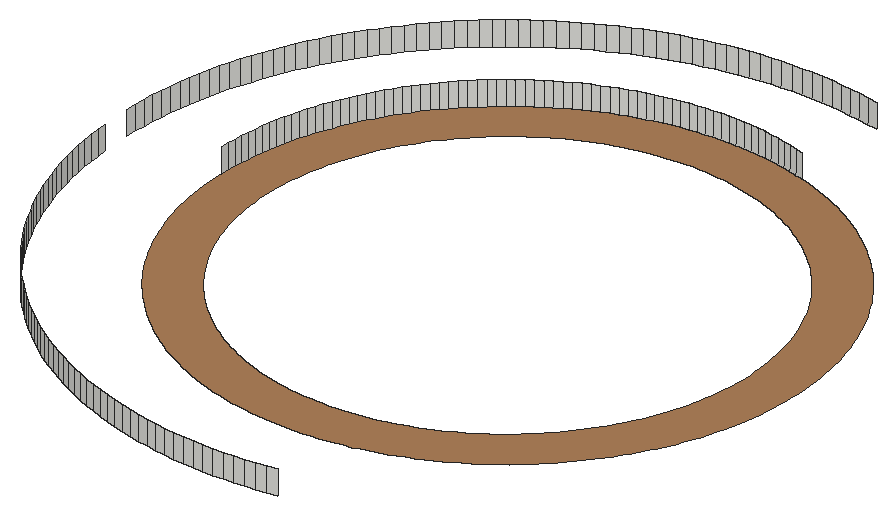
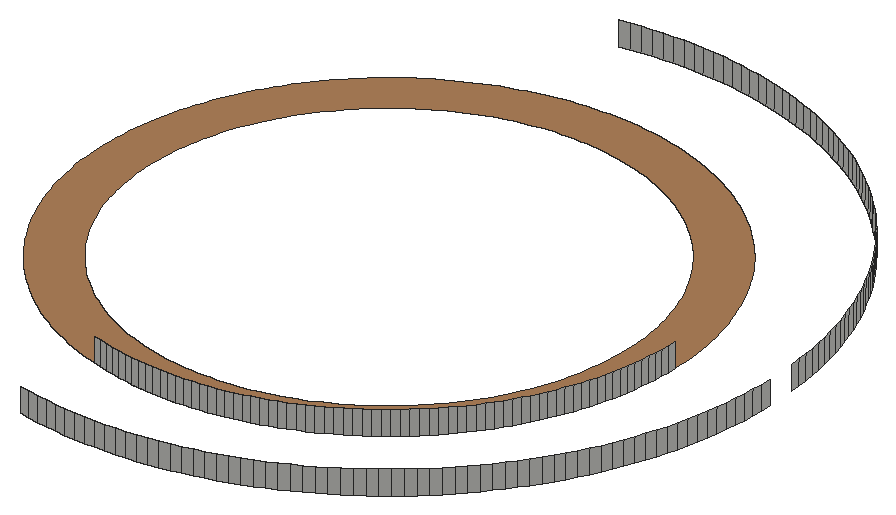
# SketchUp Ruby script. Lengths in inches.
U = 1.inch
M = Sketchup.active_model
def pt(a) = Geom::Point3d.new(a.map { |v| v * U })
def face(e, loops, mat)
  f = e.add_face(loops[0].map { |a| pt(a) })
  loops[1..].each { |l| e.add_face(l.map { |a| pt(a) }).erase! }
  f.material = f.back_material = mat if mat
  f
end
# faces: each face lists its corners as indices into pts; further lists are holes
def faces(e, pts, list, mat = nil) = list.each { |f| face(e, (f[0].is_a?(Array) ? f : [f]).map { |l| l.map { |i| pts[i] } }, mat) }
# xy, xz, yz: faces in a plane at the given z, y or x. An outline is a flat list of corners, or four numbers for a rectangle; further outlines are holes
def ring(l) = l.size == 4 ? [[l[0], l[1]], [l[2], l[1]], [l[2], l[3]], [l[0], l[3]]] : l.each_slice(2).to_a
def flat(e, list, mat, &to3) = list.each { |f| face(e, (f[0].is_a?(Array) ? f : [f]).map { |l| ring(l).map { |u, v| to3.(u, v) } }, mat) }
def xy(e, z, list, mat = nil) = flat(e, list, mat) { |x, y| [x, y, z] }
def xz(e, y, list, mat = nil) = flat(e, list, mat) { |x, z| [x, y, z] }
def yz(e, x, list, mat = nil) = flat(e, list, mat) { |y, z| [x, y, z] }
def lines(e, pts, list) = list.each { |a, b| e.add_line(pt(pts[a]), pt(pts[b])) }
# prism: a flat outline (further loops are holes) pulled along v
def prism(e, loops, v, mat = nil)
  f = face(e, loops, mat); d = Geom::Vector3d.new(v.map { |x| x * U })
  f.pushpull(f.normal.samedirection?(d) ? d.length : -d.length)
end
def box(e, o, s, mat = nil) = prism(e, [[o, [o[0] + s[0], o[1], o[2]], [o[0] + s[0], o[1] + s[1], o[2]], [o[0], o[1] + s[1], o[2]]]], [0, 0, s[2]], mat)
def at(x, y, z, deg = 0) = Geom::Transformation.translation(pt([x, y, z])) * Geom::Transformation.rotation(ORIGIN, Z_AXIS, deg.degrees)
def axes(o, x, y, z) = Geom::Transformation.new([*x, 0, *y, 0, *z, 0, *pt(o).to_a, 1])
def part(name) = M.definitions.add(name)
# library, detail: a bought-in or finely detailed component or shape, given as its bounding box
def library(name, o, s) = part(name).tap { |d| box(d.entities, o, s) }
def detail(e, o, s) = box(e.add_group.entities, o, s)
def put(e, d, t, mat = nil) = e.add_instance(d, t).tap { |i| i.material = mat if mat }
def group(e, t, mat = nil) = e.add_group.tap { |g| g.transformation = t; g.material = mat if mat }.entities
root = M.entities
M.materials.add("01 - Default1").color = [173, 128, 89]
xy(root,111.3125,[[[905.98,253.26,904.09,253.28,902.21,253.35,900.33,253.48,898.45,253.65,896.58,253.87,894.72,254.14,892.86,254.46,891.01,254.83,889.17,255.25,887.34,255.71,885.53,256.22,883.73,256.78,881.94,257.39,880.18,258.04,878.43,258.74,876.69,259.48,874.98,260.27,873.29,261.1,871.625,261.98,869.98,262.9,868.36,263.87,866.76,264.87,865.2,265.92,863.66,267.01,862.15,268.13,860.67,269.3,859.22,270.51,857.8,271.75,856.42,273.03,855.07,274.34,853.75,275.69,852.47,277.08,851.23,278.5,850.02,279.95,848.86,281.43,847.73,282.9375,846.64,284.47,845.59,286.04,844.59,287.64,843.625,289.26,842.7,290.9,841.83,292.57,840.99,294.26,840.2,295.97,839.46,297.7,838.76,299.45,838.11,301.22,837.5,303.01,836.94,304.81,836.43,306.62,835.97,308.45,835.55,310.29,835.18,312.14,834.87,313.99,834.59,315.86,834.375,317.73,834.2,319.61,834.08,321.49,834,323.37,833.98,325.26,834,327.14,834.08,329.02,834.2,330.91,834.375,332.78,834.59,334.65,834.87,336.52,835.18,338.38,835.55,340.23,835.97,342.0625,836.43,343.89,836.94,345.71,837.5,347.51,838.11,349.29,838.76,351.06,839.46,352.81,840.2,354.54,840.99,356.25,841.83,357.94,842.7,359.61,843.625,361.26,844.59,362.875,845.59,364.47,846.64,366.04,847.73,367.58,848.86,369.09,850.02,370.57,851.23,372.02,852.47,373.43,853.75,374.82,855.07,376.17,856.42,377.48,857.8,378.76,859.22,380.01,860.67,381.21,862.15,382.38,863.66,383.51,865.2,384.59,866.76,385.64,868.36,386.65,869.98,387.61,871.625,388.53,873.29,389.41,874.98,390.24,876.69,391.03,878.43,391.78,880.18,392.47,881.94,393.125,883.73,393.73,885.53,394.29,887.34,394.8,889.17,395.27,891.01,395.68,892.86,396.05,894.72,396.37,896.58,396.64,898.45,396.86,900.33,397.03,902.21,397.16,904.09,397.23,905.98,397.26,907.86,397.23,909.75,397.16,911.63,397.03,913.5,396.86,915.375,396.64,917.24,396.37,919.1,396.05,920.95,395.68,922.79,395.27,924.61,394.8,926.43,394.29,928.23,393.73,930.01,393.125,931.78,392.47,933.53,391.78,935.26,391.03,936.98,390.24,938.67,389.41,940.33,388.53,941.98,387.61,943.6,386.65,945.19,385.64,946.76,384.59,948.3,383.51,949.81,382.38,951.29,381.21,952.74,380.01,954.16,378.76,955.54,377.48,956.89,376.17,958.21,374.82,959.49,373.43,960.73,372.02,961.93,370.57,963.1,369.09,964.23,367.58,965.32,366.04,966.36,364.47,967.37,362.875,968.33,361.26,969.25,359.61,970.13,357.94,970.96,356.25,971.75,354.54,972.5,352.81,973.2,351.06,973.85,349.29,974.45,347.51,975.01,345.71,975.53,343.89,975.99,342.0625,976.41,340.23,976.77,338.38,977.09,336.52,977.36,334.65,977.58,332.78,977.76,330.91,977.88,329.02,977.95,327.14,977.98,325.26,977.95,323.37,977.88,321.49,977.76,319.61,977.58,317.73,977.36,315.86,977.09,313.99,976.77,312.14,976.41,310.29,975.99,308.45,975.53,306.62,975.01,304.81,974.45,303.01,973.85,301.22,973.2,299.45,972.5,297.7,971.75,295.97,970.96,294.26,970.13,292.57,969.25,290.9,968.33,289.26,967.37,287.64,966.36,286.04,965.32,284.47,964.23,282.9375,963.1,281.43,961.93,279.95,960.73,278.5,959.49,277.08,958.21,275.69,956.89,274.34,955.54,273.03,954.16,271.75,952.74,270.51,951.29,269.3,949.81,268.13,948.3,267.01,946.76,265.92,945.19,264.87,943.6,263.87,941.98,262.9,940.33,261.98,938.67,261.1,936.98,260.27,935.26,259.48,933.53,258.74,931.78,258.04,930.01,257.39,928.23,256.78,926.43,256.22,924.61,255.71,922.79,255.25,920.95,254.83,919.1,254.46,917.24,254.14,915.375,253.87,913.5,253.65,911.63,253.48,909.75,253.35,907.86,253.28],[905.98,265.26,907.55,265.28,909.12,265.34,910.6875,265.44,912.25,265.58,913.81,265.77,915.36,265.99,916.91,266.26,918.45,266.57,919.99,266.91,921.51,267.3,923.02,267.73,924.52,268.19,926.01,268.7,927.48,269.24,928.94,269.82,930.38,270.44,931.81,271.1,933.22,271.8,934.61,272.53,935.98,273.29,937.33,274.1,938.66,274.9375,939.96,275.81,941.25,276.72,942.5,277.66,943.74,278.63,944.95,279.63,946.125,280.67,947.28,281.73,948.41,282.83,949.5,283.95,950.57,285.11,951.6,286.29,952.61,287.5,953.58,288.73,954.52,289.99,955.43,291.27,956.3,292.58,957.14,293.91,957.94,295.26,958.71,296.625,959.4375,298.02,960.13,299.43,960.79,300.85,961.41,302.3,961.99,303.75,962.54,305.23,963.04,306.72,963.51,308.22,963.93,309.73,964.32,311.25,964.67,312.78,964.97,314.32,965.24,315.87,965.47,317.42,965.65,318.98,965.79,320.55,965.9,322.12,965.96,323.6875,965.98,325.26,965.96,326.83,965.9,328.4,965.79,329.96,965.65,331.53,965.47,333.09,965.24,334.64,964.97,336.19,964.67,337.73,964.32,339.26,963.93,340.79,963.51,342.3,963.04,343.8,962.54,345.28,961.99,346.76,961.41,348.22,960.79,349.66,960.13,351.09,959.4375,352.5,958.71,353.89,957.94,355.26,957.14,356.61,956.3,357.93,955.43,359.24,954.52,360.52,953.58,361.78,952.61,363.02,951.6,364.22,950.57,365.4,949.5,366.56,948.41,367.68,947.28,368.78,946.125,369.84,944.95,370.88,943.74,371.88,942.5,372.86,941.25,373.8,939.96,374.7,938.66,375.58,937.33,376.41,935.98,377.22,934.61,377.99,933.22,378.72,931.81,379.41,930.38,380.07,928.94,380.6875,927.48,381.27,926.01,381.81,924.52,382.32,923.02,382.79,921.51,383.21,919.99,383.6,918.45,383.95,916.91,384.25,915.36,384.52,913.81,384.74,912.25,384.93,910.6875,385.07,909.12,385.17,907.55,385.24,905.98,385.26,904.41,385.24,902.84,385.17,901.27,385.07,899.71,384.93,898.15,384.74,896.59,384.52,895.04,384.25,893.5,383.95,891.97,383.6,890.45,383.21,888.9375,382.79,887.4375,382.32,885.95,381.81,884.48,381.27,883.02,380.6875,881.57,380.07,880.15,379.41,878.74,378.72,877.35,377.99,875.98,377.22,874.63,376.41,873.3,375.58,871.99,374.7,870.71,373.8,869.45,372.86,868.22,371.88,867.01,370.88,865.83,369.84,864.68,368.78,863.55,367.68,862.46,366.56,861.39,365.4,860.35,364.22,859.35,363.02,858.38,361.78,857.4375,360.52,856.53,359.24,855.66,357.93,854.82,356.61,854.02,355.26,853.25,353.89,852.52,352.5,851.82,351.09,851.17,349.66,850.55,348.22,849.96,346.76,849.42,345.28,848.92,343.8,848.45,342.3,848.02,340.79,847.64,339.26,847.29,337.73,846.98,336.19,846.72,334.64,846.49,333.09,846.31,331.53,846.16,329.96,846.0625,328.4,846,326.83,845.98,325.26,846,323.6875,846.0625,322.12,846.16,320.55,846.31,318.98,846.49,317.42,846.72,315.87,846.98,314.32,847.29,312.78,847.64,311.25,848.02,309.73,848.45,308.22,848.92,306.72,849.42,305.23,849.96,303.75,850.55,302.3,851.17,300.85,851.82,299.43,852.52,298.02,853.25,296.625,854.02,295.26,854.82,293.91,855.66,292.58,856.53,291.27,857.4375,289.99,858.38,288.73,859.35,287.5,860.35,286.29,861.39,285.11,862.46,283.95,863.55,282.83,864.68,281.73,865.83,280.67,867.01,279.63,868.22,278.63,869.45,277.66,870.71,276.72,871.99,275.81,873.3,274.9375,874.63,274.1,875.98,273.29,877.35,272.53,878.74,271.8,880.15,271.1,881.57,270.44,883.02,269.82,884.48,269.24,885.95,268.7,887.4375,268.19,888.9375,267.73,890.45,267.3,891.97,266.91,893.5,266.57,895.04,266.26,896.59,265.99,898.15,265.77,899.71,265.58,901.27,265.44,902.84,265.34,904.41,265.28]]],"01 - Default1")
p = [[900.95,229.39,117.3125],[903.47,229.29,117.3125],[903.47,229.29,111.3125],[900.95,229.39,111.3125],[905.98,229.26,117.3125],[905.98,229.26,111.3125],
  [908.49,229.29,117.3125],[908.49,229.29,111.3125],[911,229.39,117.3125],[911,229.39,111.3125],[898.45,229.55,117.3125],[898.45,229.55,111.3125],
  [913.51,229.55,117.3125],[913.51,229.55,111.3125],[895.94,229.78,117.3125],[895.94,229.78,111.3125],[916.01,229.78,117.3125],[916.01,229.78,111.3125],
  [893.45,230.08,117.3125],[893.45,230.08,111.3125],[918.51,230.08,117.3125],[918.51,230.08,111.3125],[890.96,230.4375,117.3125],[890.96,230.4375,111.3125],
  [921,230.4375,117.3125],[921,230.4375,111.3125],[888.48,230.86,117.3125],[888.48,230.86,111.3125],[923.47,230.86,117.3125],[923.47,230.86,111.3125],
  [886.02,231.35,117.3125],[886.02,231.35,111.3125],[883.57,231.91,117.3125],[883.57,231.91,111.3125],[881.13,232.53,117.3125],[881.13,232.53,111.3125],
  [878.71,233.21,117.3125],[878.71,233.21,111.3125],[876.3125,233.95,117.3125],[876.3125,233.95,111.3125],[873.93,234.76,117.3125],[873.93,234.76,111.3125],
  [871.58,235.63,117.3125],[871.58,235.63,111.3125],[869.24,236.5625,117.3125],[869.24,236.5625,111.3125],[866.93,237.56,117.3125],[866.93,237.56,111.3125],
  [864.65,238.61,117.3125],[864.65,238.61,111.3125],[862.4,239.72,117.3125],[862.4,239.72,111.3125],[860.17,240.89,117.3125],[860.17,240.89,111.3125],
  [857.98,242.12,117.3125],[857.98,242.12,111.3125],[855.82,243.4,117.3125],[855.82,243.4,111.3125],[853.69,244.74,117.3125],[853.69,244.74,111.3125],
  [851.6,246.14,117.3125],[851.6,246.14,111.3125],[849.55,247.59,117.3125],[849.55,247.59,111.3125],[847.54,249.09,117.3125],[847.54,249.09,111.3125],
  [845.5625,250.65,117.3125],[845.5625,250.65,111.3125],[843.63,252.26,117.3125],[843.63,252.26,111.3125],[841.74,253.91,117.3125],[841.74,253.91,111.3125],
  [839.9,255.62,117.3125],[839.9,255.62,111.3125],[838.1,257.375,117.3125],[838.1,257.375,111.3125],[836.34,259.17,117.3125],[836.34,259.17,111.3125],
  [834.64,261.02,117.3125],[834.64,261.02,111.3125],[832.98,262.91,117.3125],[832.98,262.91,111.3125],[831.37,264.84,117.3125],[831.37,264.84,111.3125],
  [829.82,266.82,117.3125],[829.82,266.82,111.3125],[828.3125,268.83,117.3125],[828.3125,268.83,111.3125],[826.86,270.88,117.3125],[826.86,270.88,111.3125],
  [825.47,272.97,117.3125],[825.47,272.97,111.3125],[824.125,275.1,117.3125],[824.125,275.1,111.3125],[822.84,277.26,117.3125],[822.84,277.26,111.3125],
  [821.61,279.45,117.3125],[821.61,279.45,111.3125],[820.44,281.67,117.3125],[820.44,281.67,111.3125],[819.33,283.93,117.3125],[819.33,283.93,111.3125],
  [818.28,286.21,117.3125],[818.28,286.21,111.3125],[817.29,288.52,117.3125],[817.29,288.52,111.3125],[816.35,290.85,117.3125],[816.35,290.85,111.3125],
  [815.49,293.21,117.3125],[815.49,293.21,111.3125],[814.68,295.59,117.3125],[814.68,295.59,111.3125],[813.93,297.99,117.3125],[813.93,297.99,111.3125],
  [813.25,300.41,117.3125],[813.25,300.41,111.3125],[812.63,302.85,117.3125],[812.63,302.85,111.3125],[812.08,305.3,117.3125],[812.08,305.3,111.3125],
  [811.59,307.76,117.3125],[811.59,307.76,111.3125],[811.16,310.24,117.3125],[811.16,310.24,111.3125],[810.8,312.73,117.3125],[810.8,312.73,111.3125],
  [810.5,315.22,117.3125],[810.5,315.22,111.3125],[810.27,317.72,117.3125],[810.27,317.72,111.3125],[810.01,327.77,117.3125],[809.98,325.26,117.3125],
  [809.98,325.26,111.3125],[810.01,327.77,111.3125],[833.98,325.26,117.3125],[834,327.14,117.3125],[834,327.14,111.3125],[833.98,325.26,111.3125],
  [834.08,329.02,117.3125],[834.08,329.02,111.3125],[810.11,330.28,117.3125],[810.11,330.28,111.3125],[834.2,330.91,117.3125],[834.2,330.91,111.3125],
  [810.27,332.79,117.3125],[810.27,332.79,111.3125],[834.375,332.78,117.3125],[834.375,332.78,111.3125],[810.5,335.29,117.3125],[810.5,335.29,111.3125],
  [834.59,334.65,117.3125],[834.59,334.65,111.3125],[834.87,336.52,117.3125],[834.87,336.52,111.3125],[810.8,337.79,117.3125],[810.8,337.79,111.3125],
  [835.18,338.38,117.3125],[835.18,338.38,111.3125],[811.16,340.27,117.3125],[811.16,340.27,111.3125],[835.55,340.23,117.3125],[835.55,340.23,111.3125],
  [835.97,342.0625,117.3125],[835.97,342.0625,111.3125],[811.59,342.75,117.3125],[811.59,342.75,111.3125],[836.43,343.89,117.3125],[836.43,343.89,111.3125],
  [812.08,345.22,117.3125],[812.08,345.22,111.3125],[836.94,345.71,117.3125],[836.94,345.71,111.3125],[812.63,347.67,117.3125],[812.63,347.67,111.3125],
  [837.5,347.51,117.3125],[837.5,347.51,111.3125],[838.11,349.29,117.3125],[838.11,349.29,111.3125],[813.25,350.1,117.3125],[813.25,350.1,111.3125],
  [838.76,351.06,117.3125],[838.76,351.06,111.3125],[813.93,352.52,117.3125],[813.93,352.52,111.3125],[839.46,352.81,117.3125],[839.46,352.81,111.3125],
  [814.68,354.92,117.3125],[814.68,354.92,111.3125],[840.2,354.54,117.3125],[840.2,354.54,111.3125],[840.99,356.25,117.3125],[840.99,356.25,111.3125],
  [815.49,357.3,117.3125],[815.49,357.3,111.3125],[841.83,357.94,117.3125],[841.83,357.94,111.3125],[816.35,359.66,117.3125],[816.35,359.66,111.3125],
  [842.7,359.61,117.3125],[842.7,359.61,111.3125],[843.625,361.26,117.3125],[843.625,361.26,111.3125],[817.29,361.99,117.3125],[817.29,361.99,111.3125],
  [844.59,362.875,117.3125],[844.59,362.875,111.3125],[818.28,364.3,117.3125],[818.28,364.3,111.3125],[845.59,364.47,117.3125],[845.59,364.47,111.3125],
  [819.33,366.59,117.3125],[819.33,366.59,111.3125],[846.64,366.04,117.3125],[846.64,366.04,111.3125],[847.73,367.58,117.3125],[847.73,367.58,111.3125],
  [820.44,368.84,117.3125],[820.44,368.84,111.3125],[848.86,369.09,117.3125],[848.86,369.09,111.3125],[821.61,371.0625,117.3125],[821.61,371.0625,111.3125],
  [850.02,370.57,117.3125],[850.02,370.57,111.3125],[851.23,372.02,117.3125],[851.23,372.02,111.3125],[822.84,373.26,117.3125],[822.84,373.26,111.3125],
  [852.47,373.43,117.3125],[852.47,373.43,111.3125],[824.125,375.42,117.3125],[824.125,375.42,111.3125],[853.75,374.82,117.3125],[853.75,374.82,111.3125],
  [855.07,376.17,117.3125],[855.07,376.17,111.3125],[825.47,377.54,117.3125],[825.47,377.54,111.3125],[856.42,377.48,117.3125],[856.42,377.48,111.3125],
  [826.86,379.63,117.3125],[826.86,379.63,111.3125],[857.8,378.76,117.3125],[857.8,378.76,111.3125],[859.22,380.01,117.3125],[859.22,380.01,111.3125],
  [828.3125,381.68,117.3125],[828.3125,381.68,111.3125],[860.67,381.21,117.3125],[860.67,381.21,111.3125],[862.15,382.38,117.3125],[862.15,382.38,111.3125],
  [829.82,383.7,117.3125],[829.82,383.7,111.3125],[863.66,383.51,117.3125],[863.66,383.51,111.3125],[865.2,384.59,117.3125],[865.2,384.59,111.3125],
  [831.37,385.67,117.3125],[831.37,385.67,111.3125],[866.76,385.64,117.3125],[866.76,385.64,111.3125],[868.36,386.65,117.3125],[868.36,386.65,111.3125],
  [832.98,387.6,117.3125],[832.98,387.6,111.3125],[869.98,387.61,117.3125],[869.98,387.61,111.3125],[834.64,389.49,117.3125],[834.64,389.49,111.3125],
  [871.625,388.53,117.3125],[871.625,388.53,111.3125],[873.29,389.41,117.3125],[873.29,389.41,111.3125],[874.98,390.24,117.3125],[874.98,390.24,111.3125],
  [836.34,391.34,117.3125],[836.34,391.34,111.3125],[876.69,391.03,117.3125],[876.69,391.03,111.3125],[878.43,391.78,117.3125],[878.43,391.78,111.3125],
  [838.1,393.14,117.3125],[838.1,393.14,111.3125],[880.18,392.47,117.3125],[880.18,392.47,111.3125],[881.94,393.125,117.3125],[881.94,393.125,111.3125],
  [839.9,394.89,117.3125],[839.9,394.89,111.3125],[883.73,393.73,117.3125],[883.73,393.73,111.3125],[885.53,394.29,117.3125],[885.53,394.29,111.3125],
  [887.34,394.8,117.3125],[887.34,394.8,111.3125],[889.17,395.27,117.3125],[889.17,395.27,111.3125],[922.79,395.27,117.3125],[924.61,394.8,117.3125],
  [924.61,394.8,111.3125],[922.79,395.27,111.3125],[841.74,396.6,117.3125],[841.74,396.6,111.3125],[891.01,395.68,117.3125],[891.01,395.68,111.3125],
  [920.95,395.68,117.3125],[920.95,395.68,111.3125],[892.86,396.05,117.3125],[892.86,396.05,111.3125],[919.1,396.05,117.3125],[919.1,396.05,111.3125],
  [894.72,396.37,117.3125],[894.72,396.37,111.3125],[917.24,396.37,117.3125],[917.24,396.37,111.3125],[896.58,396.64,117.3125],[896.58,396.64,111.3125],
  [915.375,396.64,117.3125],[915.375,396.64,111.3125],[843.63,398.26,117.3125],[843.63,398.26,111.3125],[898.45,396.86,117.3125],[898.45,396.86,111.3125],
  [913.5,396.86,117.3125],[913.5,396.86,111.3125],[900.33,397.03,117.3125],[900.33,397.03,111.3125],[911.63,397.03,117.3125],[911.63,397.03,111.3125],
  [902.21,397.16,117.3125],[902.21,397.16,111.3125],[909.75,397.16,117.3125],[909.75,397.16,111.3125],[904.09,397.23,117.3125],[904.09,397.23,111.3125],
  [905.98,397.26,117.3125],[905.98,397.26,111.3125],[907.86,397.23,117.3125],[907.86,397.23,111.3125],[845.5625,399.86,117.3125],[845.5625,399.86,111.3125],
  [847.54,401.42,117.3125],[847.54,401.42,111.3125],[849.55,402.92,117.3125],[849.55,402.92,111.3125],[851.6,404.37,117.3125],[851.6,404.37,111.3125],
  [853.69,405.77,117.3125],[853.69,405.77,111.3125],[855.82,407.11,117.3125],[855.82,407.11,111.3125],[857.98,408.39,117.3125],[857.98,408.39,111.3125],
  [860.17,409.62,117.3125],[860.17,409.62,111.3125],[862.4,410.79,117.3125],[862.4,410.79,111.3125],[864.65,411.9,117.3125],[864.65,411.9,111.3125],
  [866.93,412.96,117.3125],[866.93,412.96,111.3125],[869.24,413.95,117.3125],[869.24,413.95,111.3125],[871.58,414.88,117.3125],[871.58,414.88,111.3125],
  [873.93,415.75,117.3125],[873.93,415.75,111.3125],[876.3125,416.56,117.3125],[876.3125,416.56,111.3125],[878.71,417.3,117.3125],[878.71,417.3,111.3125],
  [881.13,417.99,117.3125],[881.13,417.99,111.3125],[883.57,418.6,117.3125],[883.57,418.6,111.3125],[886.02,419.16,117.3125],[886.02,419.16,111.3125],
  [888.48,419.65,117.3125],[888.48,419.65,111.3125],[890.96,420.07,117.3125],[890.96,420.07,111.3125],[923.47,419.65,117.3125],[921,420.07,117.3125],
  [921,420.07,111.3125],[923.47,419.65,111.3125],[893.45,420.43,117.3125],[893.45,420.43,111.3125],[918.51,420.43,117.3125],[918.51,420.43,111.3125],
  [895.94,420.73,117.3125],[895.94,420.73,111.3125],[916.01,420.73,117.3125],[916.01,420.73,111.3125],[898.45,420.96,117.3125],[898.45,420.96,111.3125],
  [913.51,420.96,117.3125],[913.51,420.96,111.3125],[900.95,421.125,117.3125],[900.95,421.125,111.3125],[911,421.125,117.3125],[911,421.125,111.3125],
  [903.47,421.22,117.3125],[903.47,421.22,111.3125],[908.49,421.22,117.3125],[908.49,421.22,111.3125],[905.98,421.26,117.3125],[905.98,421.26,111.3125]]
faces(root,p,[[0,1,2,3],[1,4,5,2],[4,6,7,5],[6,8,9,7],[10,0,3,11],[8,12,13,9],[14,10,11,15],[12,16,17,13],
  [18,14,15,19],[16,20,21,17],[22,18,19,23],[20,24,25,21],[26,22,23,27],[24,28,29,25],[30,26,27,31],[32,30,31,33],
  [34,32,33,35],[36,34,35,37],[38,36,37,39],[40,38,39,41],[42,40,41,43],[44,42,43,45],[46,44,45,47],[48,46,47,49],
  [50,48,49,51],[52,50,51,53],[54,52,53,55],[56,54,55,57],[58,56,57,59],[60,58,59,61],[62,60,61,63],[64,62,63,65],
  [66,64,65,67],[68,66,67,69],[70,68,69,71],[72,70,71,73],[74,72,73,75],[76,74,75,77],[78,76,77,79],[80,78,79,81],
  [82,80,81,83],[84,82,83,85],[86,84,85,87],[88,86,87,89],[90,88,89,91],[92,90,91,93],[94,92,93,95],[96,94,95,97],
  [98,96,97,99],[100,98,99,101],[102,100,101,103],[104,102,103,105],[106,104,105,107],[108,106,107,109],[110,108,109,111],[112,110,111,113],
  [114,112,113,115],[116,114,115,117],[118,116,117,119],[120,118,119,121],[122,120,121,123],[124,122,123,125],[126,124,125,127],[128,126,127,129],
  [130,131,132,133],[134,135,136,137],[135,138,139,136],[140,130,133,141],[138,142,143,139],[144,140,141,145],[142,146,147,143],[148,144,145,149],
  [146,150,151,147],[150,152,153,151],[154,148,149,155],[152,156,157,153],[158,154,155,159],[156,160,161,157],[160,162,163,161],[164,158,159,165],
  [162,166,167,163],[168,164,165,169],[166,170,171,167],[172,168,169,173],[170,174,175,171],[174,176,177,175],[178,172,173,179],[176,180,181,177],
  [182,178,179,183],[180,184,185,181],[186,182,183,187],[184,188,189,185],[188,190,191,189],[192,186,187,193],[190,194,195,191],[196,192,193,197],
  [194,198,199,195],[198,200,201,199],[202,196,197,203],[200,204,205,201],[206,202,203,207],[204,208,209,205],[210,206,207,211],[208,212,213,209],
  [212,214,215,213],[216,210,211,217],[214,218,219,215],[220,216,217,221],[218,222,223,219],[222,224,225,223],[226,220,221,227],[224,228,229,225],
  [230,226,227,231],[228,232,233,229],[232,234,235,233],[236,230,231,237],[234,238,239,235],[240,236,237,241],[238,242,243,239],[242,244,245,243],
  [246,240,241,247],[244,248,249,245],[248,250,251,249],[252,246,247,253],[250,254,255,251],[254,256,257,255],[258,252,253,259],[256,260,261,257],
  [260,262,263,261],[264,258,259,265],[262,266,267,263],[268,264,265,269],[266,270,271,267],[270,272,273,271],[272,274,275,273],[276,268,269,277],
  [274,278,279,275],[278,280,281,279],[282,276,277,283],[280,284,285,281],[284,286,287,285],[288,282,283,289],[286,290,291,287],[290,292,293,291],
  [292,294,295,293],[294,296,297,295],[298,299,300,301],[302,288,289,303],[296,304,305,297],[306,298,301,307],[304,308,309,305],[310,306,307,311],
  [308,312,313,309],[314,310,311,315],[312,316,317,313],[318,314,315,319],[320,302,303,321],[316,322,323,317],[324,318,319,325],[322,326,327,323],
  [328,324,325,329],[326,330,331,327],[332,328,329,333],[330,334,335,331],[334,336,337,335],[336,338,339,337],[338,332,333,339],[340,320,321,341],
  [342,340,341,343],[344,342,343,345],[346,344,345,347],[348,346,347,349],[350,348,349,351],[352,350,351,353],[354,352,353,355],[356,354,355,357],
  [358,356,357,359],[360,358,359,361],[362,360,361,363],[364,362,363,365],[366,364,365,367],[368,366,367,369],[370,368,369,371],[372,370,371,373],
  [374,372,373,375],[376,374,375,377],[378,376,377,379],[380,378,379,381],[382,383,384,385],[386,380,381,387],[383,388,389,384],[390,386,387,391],
  [388,392,393,389],[394,390,391,395],[392,396,397,393],[398,394,395,399],[396,400,401,397],[402,398,399,403],[400,404,405,401],[406,402,403,407],
  [404,406,407,405]])
